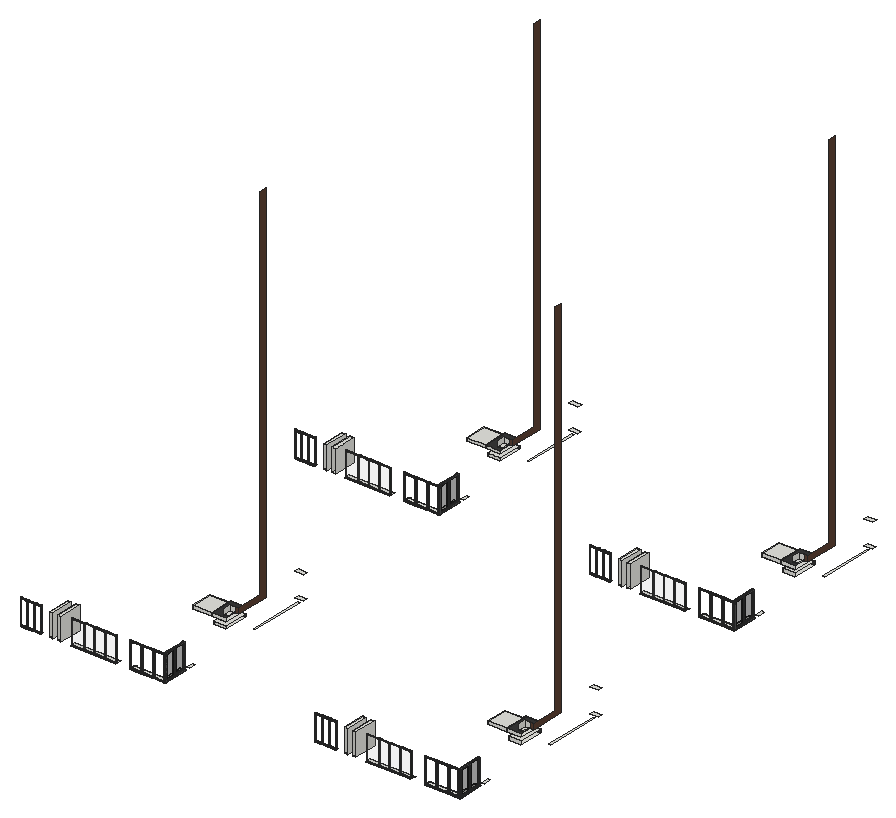
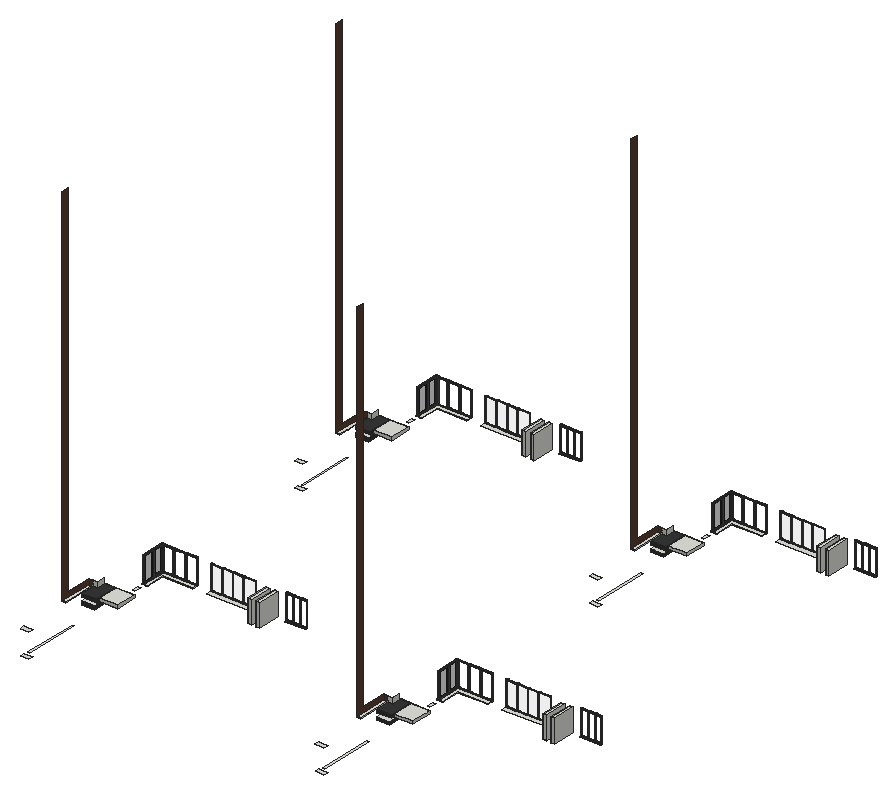
# SketchUp Ruby script. Lengths in inches.
U = 1.inch
M = Sketchup.active_model
def pt(a) = Geom::Point3d.new(a.map { |v| v * U })
def face(e, loops, mat)
  f = e.add_face(loops[0].map { |a| pt(a) })
  loops[1..].each { |l| e.add_face(l.map { |a| pt(a) }).erase! }
  f.material = f.back_material = mat if mat
  f
end
# faces: each face lists its corners as indices into pts; further lists are holes
def faces(e, pts, list, mat = nil) = list.each { |f| face(e, (f[0].is_a?(Array) ? f : [f]).map { |l| l.map { |i| pts[i] } }, mat) }
# xy, xz, yz: faces in a plane at the given z, y or x. An outline is a flat list of corners, or four numbers for a rectangle; further outlines are holes
def ring(l) = l.size == 4 ? [[l[0], l[1]], [l[2], l[1]], [l[2], l[3]], [l[0], l[3]]] : l.each_slice(2).to_a
def flat(e, list, mat, &to3) = list.each { |f| face(e, (f[0].is_a?(Array) ? f : [f]).map { |l| ring(l).map { |u, v| to3.(u, v) } }, mat) }
def xy(e, z, list, mat = nil) = flat(e, list, mat) { |x, y| [x, y, z] }
def xz(e, y, list, mat = nil) = flat(e, list, mat) { |x, z| [x, y, z] }
def yz(e, x, list, mat = nil) = flat(e, list, mat) { |y, z| [x, y, z] }
def lines(e, pts, list) = list.each { |a, b| e.add_line(pt(pts[a]), pt(pts[b])) }
# prism: a flat outline (further loops are holes) pulled along v
def prism(e, loops, v, mat = nil)
  f = face(e, loops, mat); d = Geom::Vector3d.new(v.map { |x| x * U })
  f.pushpull(f.normal.samedirection?(d) ? d.length : -d.length)
end
def box(e, o, s, mat = nil) = prism(e, [[o, [o[0] + s[0], o[1], o[2]], [o[0] + s[0], o[1] + s[1], o[2]], [o[0], o[1] + s[1], o[2]]]], [0, 0, s[2]], mat)
def at(x, y, z, deg = 0) = Geom::Transformation.translation(pt([x, y, z])) * Geom::Transformation.rotation(ORIGIN, Z_AXIS, deg.degrees)
def axes(o, x, y, z) = Geom::Transformation.new([*x, 0, *y, 0, *z, 0, *pt(o).to_a, 1])
def part(name) = M.definitions.add(name)
# library, detail: a bought-in or finely detailed component or shape, given as its bounding box
def library(name, o, s) = part(name).tap { |d| box(d.entities, o, s) }
def detail(e, o, s) = box(e.add_group.entities, o, s)
def put(e, d, t, mat = nil) = e.add_instance(d, t).tap { |i| i.material = mat if mat }
def group(e, t, mat = nil) = e.add_group.tap { |g| g.transformation = t; g.material = mat if mat }.entities
root = M.entities
M.materials.add("Glass_Tinted_Gray").color = [0, 0, 0]
M.materials["Glass_Tinted_Gray"].alpha = 0.125
M.materials.add("Glazing").color = [128, 128, 128]
M.materials["Glazing"].alpha = 0.05
M.materials.add("Powdercoating").color = [41, 44, 40]
M.materials.add("Wine2").color = [0, 0, 0]
M.materials["Wine2"].alpha = 0
M.materials.add("[0130_Gainsboro]").color = [39, 45, 50]
M.materials.add("[0135_DarkGray]").color = [81, 81, 81]
M.materials.add("[Granite Brown]1").color = [89, 63, 50]
M.materials.add("[Mirror 02]").color = [229, 229, 229]
M.materials.add("[Slate Light Tile]").color = [54, 54, 54]
M.materials.add("[Terrazzo Light Blue]").color = [196, 214, 227]
c1 = part("Framed glazing panel")
xy(c1.entities,0,[[0,-0.98,43.07,0],[0,0,43.07,1.4]],"[0130_Gainsboro]")
xy(c1.entities,0.3,[[0.3,-1.43,42.77,-0.98]],"[0130_Gainsboro]")
xy(c1.entities,2.95,[[2.95,-1.43,40.12,-0.63],[2.95,-0.63,40.12,0],[2.95,0,40.12,0.64],[2.95,0.64,40.12,1.4]],"[0130_Gainsboro]")
xy(c1.entities,3.54,[[3.54,-0.63,39.53,0],[3.54,0,39.53,0.64]],"[0130_Gainsboro]")
xy(c1.entities,111.8125,[[3.54,-0.63,39.53,0],[3.54,0,39.53,0.64]],"[0130_Gainsboro]")
xy(c1.entities,112.4,[[2.95,-1.43,40.12,-0.63],[2.95,-0.63,40.12,0],[2.95,0,40.12,0.64],[2.95,0.64,40.12,1.4]],"[0130_Gainsboro]")
xy(c1.entities,115.05,[[0.3,-1.43,42.77,-0.98]],"[0130_Gainsboro]")
xy(c1.entities,115.35,[[0,-0.98,43.07,0],[0,0,43.07,1.4]],"[0130_Gainsboro]")
xz(c1.entities,-1.43,[[[0.3,0.3,42.77,115.05],[2.95,2.95,40.12,112.4]]],"[0130_Gainsboro]")
xz(c1.entities,-0.98,[[[0,0,43.07,115.35],[0.3,0.3,42.77,115.05]]],"[0130_Gainsboro]")
xz(c1.entities,-0.63,[[[2.95,2.95,40.12,112.4],[3.54,3.54,39.53,111.8125]]],"[0130_Gainsboro]")
xz(c1.entities,0,[[3.54,3.54,39.53,111.8125]],"Wine2")
xz(c1.entities,0,[[[0,0,43.07,115.35],[2.95,2.95,40.12,112.4]],[[2.95,2.95,40.12,112.4],[3.54,3.54,39.53,111.8125]]],"[0130_Gainsboro]")
xz(c1.entities,0.64,[[[2.95,2.95,40.12,112.4],[3.54,3.54,39.53,111.8125]]],"[0130_Gainsboro]")
xz(c1.entities,1.4,[[[0,0,43.07,115.35],[2.95,2.95,40.12,112.4]]],"[0130_Gainsboro]")
yz(c1.entities,0,[[-0.98,0,0,115.35],[0,0,1.4,115.35]],"[0130_Gainsboro]")
yz(c1.entities,0.3,[[-1.43,0.3,-0.98,115.05]],"[0130_Gainsboro]")
yz(c1.entities,2.95,[[-1.43,2.95,-0.63,112.4],[-0.63,2.95,0,112.4],[0,2.95,0.64,112.4],[0.64,2.95,1.4,112.4]],"[0130_Gainsboro]")
yz(c1.entities,3.54,[[-0.63,3.54,0,111.8125],[0,3.54,0.64,111.8125]],"[0130_Gainsboro]")
yz(c1.entities,39.53,[[-0.63,3.54,0,111.8125],[0,3.54,0.64,111.8125]],"[0130_Gainsboro]")
yz(c1.entities,40.12,[[-1.43,2.95,-0.63,112.4],[-0.63,2.95,0,112.4],[0,2.95,0.64,112.4],[0.64,2.95,1.4,112.4]],"[0130_Gainsboro]")
yz(c1.entities,42.77,[[-1.43,0.3,-0.98,115.05]],"[0130_Gainsboro]")
yz(c1.entities,43.07,[[-0.98,0,0,115.35],[0,0,1.4,115.35]],"[0130_Gainsboro]")
c2 = part("Glazed panel assembly")
put(c2.entities,c1,axes([90.57,1.43,0],[1.05148,0,0],[0,1,0],[0,0,1]))
put(c2.entities,c1,axes([0,1.43,0],[1.05148,0,0],[0,1,0],[0,0,1]))
put(c2.entities,c1,axes([45.29,1.43,0],[1.05148,0,0],[0,1,0],[0,0,1]))
c3 = part("PENTEK_RP Fineline 50S_Sliding_DoorCase_E1")
box(c3.entities,[0,0,0],[1.51,3.66,99.27],"[0135_DarkGray]")
c4 = part("PENTEK_RP Fineline 50S_SlidingDooe_Case_E2")
box(c4.entities,[0,0,0],[96.25,3.66,1.51],"[0135_DarkGray]")
c5 = part("pentek_RP Fineline 50S_SlidingDoor_Case")
put(c5.entities,c3,at(97.76,0,0))
put(c5.entities,c4,at(1.51,0,0))
put(c5.entities,c3,at(0,0,0))
put(c5.entities,c4,at(1.51,0,97.76))
c6 = part("PENTEK_RP Fineline 50S_SlidingDoor_GlazingBead_2")
box(c6.entities,[0,0,0],[0.56,0.59,94.39],"[0135_DarkGray]")
c7 = part("PENTEK_RP Fineline 50S_SlidingDoor_Glass")
box(c7.entities,[0,0,0],[46.58,0.16,94.39],"Glass_Tinted_Gray")
c8 = part("PENTEK_RP Fineline 50S_SlidingDoor_GlazingBead")
box(c8.entities,[0,0,0],[45.47,0.59,0.56],"[0135_DarkGray]")
c9 = part("PENTEK_RP Fineline 50S_SlidingDoor_Leaf_E1")
xy(c9.entities,0,[[0,0,0.93,1.97],[0.93,1.57,1.49,1.97]],"[0135_DarkGray]")
xy(c9.entities,96.25,[[0,0,0.93,0,0.93,1.57,1.49,1.57,1.49,1.97,0,1.97]],"[0135_DarkGray]")
xz(c9.entities,0,[[0,0,0.93,96.25]],"[0135_DarkGray]")
xz(c9.entities,1.57,[[0.93,0,1.49,95.32],[0.93,95.32,1.49,96.25]],"[0135_DarkGray]")
xz(c9.entities,1.97,[[0,0,1.49,96.25]],"[0135_DarkGray]")
yz(c9.entities,0,[[0,0,1.97,96.25]],"[0135_DarkGray]")
yz(c9.entities,0.93,[[0,0,1.57,0.93],[0,0.93,1.57,95.32],[0,95.32,1.57,96.25]],"[0135_DarkGray]")
yz(c9.entities,1.49,[[1.57,0,1.97,95.32],[1.57,95.32,1.97,96.25]],"[0135_DarkGray]")
c10 = part("PENTEK_RP Fineline 50S_SlidingDoor_Leaf_E2")
xy(c10.entities,0,[[0,0,0,1.57,0.56,1.57,0.56,1.97,46.02,1.97,46.02,1.57,46.58,1.57,46.58,0]],"[0135_DarkGray]")
xy(c10.entities,0.93,[[0,0,46.58,1.57]],"[0135_DarkGray]")
xy(c10.entities,1.49,[[0.56,1.57,46.02,1.97]],"[0135_DarkGray]")
xz(c10.entities,0,[[0,0,46.58,0.93]],"[0135_DarkGray]")
xz(c10.entities,1.57,[[0,0,0.56,0.93],[46.02,0,46.58,0.93],[0.56,0.93,46.02,1.49]],"[0135_DarkGray]")
xz(c10.entities,1.97,[[0.56,0,46.02,1.49]],"[0135_DarkGray]")
yz(c10.entities,0,[[0,0,1.57,0.93]],"[0135_DarkGray]")
yz(c10.entities,0.56,[[1.57,0,1.97,0.93],[1.57,0.93,1.97,1.49]],"[0135_DarkGray]")
yz(c10.entities,46.02,[[1.57,0,1.97,0.93],[1.57,0.93,1.97,1.49]],"[0135_DarkGray]")
yz(c10.entities,46.58,[[0,0,1.57,0.93]],"[0135_DarkGray]")
c11 = part("PENTEK_RP Fineline S_SlidingDoor_Leaf1")
put(c11.entities,c6,at(0.93,0,0.93))
put(c11.entities,c6,at(46.96,0,0.93))
put(c11.entities,c7,at(1.49,1.42,0.93))
put(c11.entities,c8,at(1.49,0,0.93))
put(c11.entities,c7,at(1.49,0.59,0.93),"[Terrazzo Light Blue]")
put(c11.entities,c9,at(0,0,0))
put(c11.entities,c9,axes([48.44,0,0],[-1,0,0],[0,1,0],[0,0,1]))
put(c11.entities,c10,axes([0.93,0,96.25],[1,0,0],[0,1,0],[0,0,-1]))
put(c11.entities,c10,at(0.93,0,0))
put(c11.entities,c8,at(1.49,0,94.77))
c12 = part("PENTEK_RP Fineline 50S_SlidingDoor_Leaf2")
put(c12.entities,c7,at(1.49,1.42,0.93))
put(c12.entities,c8,at(1.49,0,94.77))
put(c12.entities,c6,at(46.96,0,0.93))
put(c12.entities,c7,at(1.49,0.59,0.93),"[Mirror 02]")
put(c12.entities,c6,at(0.93,0,0.93))
put(c12.entities,c9,at(0,0,0))
put(c12.entities,c9,axes([48.44,0,0],[-1,0,0],[0,1,0],[0,0,1]))
put(c12.entities,c8,at(1.49,0,0.93))
put(c12.entities,c10,axes([0.93,0,96.25],[1,0,0],[0,1,0],[0,0,-1]))
put(c12.entities,c10,at(0.93,0,0))
c13 = part("PENTEK - Slimmest Steel Sliding Door / Window\#1")
put(c13.entities,c5,at(0,-1.88,-0.09))
put(c13.entities,c11,at(1.51,-2.27,1.42))
put(c13.entities,c12,at(49.32,-0.3,1.42))
c14 = part("Group\#15")
xy(c14.entities,0,[[0,-55.94,0.71,45.94]])
xy(c14.entities,0.2,[[0,-55.94,0.47,45.94],[0.47,45.94,0.71,46.42]])
xy(c14.entities,2.36,[[0.47,-55.94,0.71,46.42]])
xz(c14.entities,-55.94,[[0,0,0.71,0,0.71,2.36,0.47,2.36,0.47,0.2,0,0.2]])
xz(c14.entities,45.94,[[0,0,0.71,0.2]])
xz(c14.entities,46.42,[[0.47,0.2,0.71,2.36]])
yz(c14.entities,0,[[-55.94,0,45.94,0.2]])
yz(c14.entities,0.47,[[-55.94,0.2,46.42,2.36]])
yz(c14.entities,0.71,[[-55.94,0,45.94,0,45.94,0.2,46.42,0.2,46.42,2.36,-55.94,2.36]])
c15 = part("Group\#7")
xy(c15.entities,0,[[0,-59.09,0.71,45.94]])
xy(c15.entities,0.2,[[0,-59.09,0.47,45.94],[0.47,45.94,0.71,46.42]])
xy(c15.entities,2.36,[[0.47,-59.09,0.71,46.42]])
xz(c15.entities,-59.09,[[0,0,0.71,0,0.71,2.36,0.47,2.36,0.47,0.2,0,0.2]])
xz(c15.entities,45.94,[[0,0,0.71,0.2]])
xz(c15.entities,46.42,[[0.47,0.2,0.71,2.36]])
yz(c15.entities,0,[[-59.09,0,45.94,0.2]])
yz(c15.entities,0.47,[[-59.09,0.2,46.42,2.36]])
yz(c15.entities,0.71,[[-59.09,0,45.94,0,45.94,0.2,46.42,0.2,46.42,2.36,-59.09,2.36]])
c16 = part("Group\#16")
prism(c16.entities,[[[0.47,-56.18,0.2],[0,-56.18,0.2],[0,-56.18,0],[0.71,-56.18,0],[0.71,-56.18,2.36],[0.47,-56.18,2.36]]],[0,28.68,0])
c17 = part("Group\#10")
box(c17.entities,[-0.73,0,0],[27.99,0.55,102.05])
c18 = part("Group\#18")
xy(c18.entities,0,[[0.47,-56.18,0.47,-55.47,0,-55.47,0,-28.21,1.18,-28.21,1.18,-56.18]])
xy(c18.entities,0.2,[[0.71,-56.18,1.18,-28.21],[0,-55.47,0.47,-28.21],[0.47,-28.21,0.71,-27.74]])
xy(c18.entities,2.36,[[0.47,-56.18,0.71,-27.74]])
xz(c18.entities,-56.18,[[0.47,0,1.18,0,1.18,0.2,0.71,0.2,0.71,2.36,0.47,2.36]])
xz(c18.entities,-55.47,[[0,0,0.47,0.2]])
xz(c18.entities,-28.21,[[0,0,1.18,0.2]])
xz(c18.entities,-27.74,[[0.47,0.2,0.71,2.36]])
yz(c18.entities,0,[[-55.47,0,-28.21,0.2]])
yz(c18.entities,0.47,[[-56.18,0,-55.47,0.2],[-56.18,0.2,-27.74,2.36]])
yz(c18.entities,0.71,[[-56.18,0.2,-27.74,2.36]])
yz(c18.entities,1.18,[[-56.18,0,-28.21,0.2]])
c19 = part("Group\#34")
xy(c19.entities,0,[[-20.45,0,7.76,1.22]])
xy(c19.entities,0.06,[[-20.39,0.06,7.7,1.22]])
xy(c19.entities,0.47,[[-19.98,0,7.28,0.06]])
xy(c19.entities,101.89,[[-19.98,0,7.28,0.06]])
xy(c19.entities,102.3,[[-20.39,0.06,7.7,1.22]])
xy(c19.entities,102.36,[[-20.45,0,7.76,1.22]])
xz(c19.entities,0,[[[-20.45,0,7.76,102.36],[-19.98,0.47,7.28,101.89]]])
xz(c19.entities,0.06,[[[-20.39,0.06,7.7,102.3],[-19.98,0.47,7.28,101.89]]])
xz(c19.entities,1.22,[[[-20.45,0,7.76,102.36],[-20.39,0.06,7.7,102.3]]])
yz(c19.entities,-20.45,[[0,0,1.22,102.36]])
yz(c19.entities,-20.39,[[0.06,0.06,1.22,102.3]])
yz(c19.entities,-19.98,[[0,0.47,0.06,101.89]])
yz(c19.entities,7.28,[[0,0.47,0.06,101.89]])
yz(c19.entities,7.7,[[0.06,0.06,1.22,102.3]])
yz(c19.entities,7.76,[[0,0,1.22,102.36]])
c20 = part("Group\#6")
put(c20.entities,c14,axes([27.97,0,7.875],[1,0,0],[0,0,-1],[0,1,0]),"Powdercoating")
put(c20.entities,c15,axes([0.71,0,6.8],[-1,0,0],[0,0,-0.97687],[0,1,0]),"Powdercoating")
put(c20.entities,c16,axes([-27.5,0,-38.07],[0,0,-1],[-1,0,0],[0,1,0]),"Powdercoating")
put(c20.entities,c17,at(1.12,0.35,-38.39),"Glazing")
put(c20.entities,c18,axes([-27.5,0,63.35],[0,0,1],[-1,0,0],[0,1,0]),"Powdercoating")
put(c20.entities,c19,at(20.6875,1.0625,-38.54),"Powdercoating")
c21 = part("Sliding door assembly")
put(c21.entities,c20,at(-1.18,4.5,38.86))
g1 = group(c21.entities,at(84.74,4.5,38.86))
put(g1,c14,axes([-27.97,0,7.875],[-1,0,0],[0,0,-1],[0,1,0]),"Powdercoating")
put(g1,c15,axes([-0.71,0,6.8],[1,0,0],[0,0,-0.97687],[0,1,0]),"Powdercoating")
put(g1,c16,axes([27.5,0,-38.07],[0,0,-1],[1,0,0],[0,1,0]),"Powdercoating")
put(g1,c17,axes([-1.12,0.35,-38.39],[-1,0,0],[0,1,0],[0,0,1]),"Glazing")
put(g1,c18,axes([27.5,0,63.35],[0,0,1],[1,0,0],[0,1,0]),"Powdercoating")
put(g1,c19,axes([-20.6875,1.0625,-38.54],[-1,0,0],[0,1,0],[0,0,1]),"Powdercoating")
g2 = group(c21.entities,at(56.0625,4.5,38.86))
put(g2,c14,axes([-27.97,0,7.875],[-1,0,0],[0,0,-1],[0,1,0]),"Powdercoating")
put(g2,c16,axes([27.5,0,-38.07],[0,0,-1],[1,0,0],[0,1,0]),"Powdercoating")
put(g2,c17,axes([-1.12,0.35,-38.39],[-1,0,0],[0,1,0],[0,0,1]),"Glazing")
put(g2,c18,axes([27.5,0,63.35],[0,0,1],[1,0,0],[0,1,0]),"Powdercoating")
put(g2,c19,axes([-20.6875,1.0625,-38.54],[-1,0,0],[0,1,0],[0,0,1]),"Powdercoating")
g3 = group(g2,at(-0.71,0,6.8),"Powdercoating")
xy(g3,-45.34,[[0.47,0.2,0.71,2.36]])
xy(g3,-44.88,[[0,0,0.71,0.2]])
xy(g3,57.73,[[0,0,0.71,0,0.71,2.36,0.47,2.36,0.47,0.2,0,0.2]])
xz(g3,0,[[0,-44.88,0.71,57.73]])
xz(g3,0.2,[[0.47,-45.34,0.71,-44.88],[0,-44.88,0.47,57.73]])
xz(g3,2.36,[[0.47,-45.34,0.71,57.73]])
yz(g3,0,[[0,-44.88,0.2,57.73]])
yz(g3,0.47,[[0.2,-45.34,2.36,57.73]])
yz(g3,0.71,[[0.2,-45.34,2.36,-45.34,2.36,57.73,0,57.73,0,-44.88,0.2,-44.88]])
put(c21.entities,c20,axes([-33.94,4.5,38.86],[1.14218,0,0],[0,1,0],[0,0,1]))
c22 = part("sliding door")
put(c22.entities,c21,at(0,-4.5,-0.08))
prism(root,[[[2132.0625,1799.9375,145.375],[1985.38,1799.9375,145.375],[1985.38,1822.9375,145.375],[2109.0625,1822.9375,145.375],[2109.0625,1902.66,145.375],[2132.0625,1902.66,145.375]]],[0,0,1.75])
prism(root,[[[913.875,1799.9375,145.375],[767.19,1799.9375,145.375],[767.19,1822.9375,145.375],[890.875,1822.9375,145.375],[890.875,1902.66,145.375],[913.875,1902.66,145.375]]],[0,0,1.75])
prism(root,[[[2132.0625,3214.625,145.375],[1985.38,3214.625,145.375],[1985.38,3237.625,145.375],[2109.0625,3237.625,145.375],[2109.0625,3317.34,145.375],[2132.0625,3317.34,145.375]]],[0,0,1.75])
prism(root,[[[913.875,3214.625,145.375],[767.19,3214.625,145.375],[767.19,3237.625,145.375],[890.875,3237.625,145.375],[890.875,3317.34,145.375],[913.875,3317.34,145.375]]],[0,0,1.75])
xy(root,145.375,[[319.53,1799.9375,399.88,1807.625],[523.04,1799.9375,709.87,1822.9375],[1537.72,1799.9375,1618.07,1807.625],[1741.23,1799.9375,1928.05,1822.9375],[902.375,1926.07,913.875,1953.7],
  [2120.5625,1926.07,2132.0625,1953.7],[913.875,2258.18,921.125,2483.21],[2132.0625,2258.18,2139.3125,2483.21],[890.875,2497.47,927.0625,2514.84],[2109.0625,2497.47,2145.25,2514.84],
  [319.53,3214.625,399.88,3222.3125],[523.04,3214.625,709.87,3237.625],[1537.72,3214.625,1618.07,3222.3125],[1741.23,3214.625,1928.05,3237.625],[902.375,3340.76,913.875,3368.39],
  [2120.5625,3340.76,2132.0625,3368.39],[913.875,3672.87,921.125,3897.9],[2132.0625,3672.87,2139.3125,3897.9],[890.875,3912.16,927.0625,3929.52],[2109.0625,3912.16,2145.25,3929.52]])
xy(root,145.8125,[[434.43,1799.9375,450.49,1893.25],[1652.62,1799.9375,1668.68,1893.25],[434.43,3214.625,450.49,3307.9375],[1652.62,3214.625,1668.68,3307.9375]])
xy(root,147.29,[[467.98,1799.9375,483.79,1893.25],[1686.17,1799.9375,1701.98,1893.25],[467.98,3214.625,483.79,3307.9375],[1686.17,3214.625,1701.98,3307.9375]])
xy(root,206.6875,[[861.3125,2113.57,913.875,2213.62],[2079.5,2113.57,2132.0625,2213.62],[861.3125,3528.25,913.875,3628.31],[2079.5,3528.25,2132.0625,3628.31]])
xy(root,220.18,[[861.3125,2113.57,913.875,2213.62],[2079.5,2113.57,2132.0625,2213.62],[861.3125,3528.25,913.875,3628.31],[2079.5,3528.25,2132.0625,3628.31]])
xy(root,234.11,[[776.875,2113.57,853.875,2200.82],[853.875,2113.57,913.875,2213.62],[1995.0625,2113.57,2072.0625,2200.82],[2072.0625,2113.57,2132.0625,2213.62],[776.875,3528.25,853.875,3615.5],
  [853.875,3528.25,913.875,3628.31],[1995.0625,3528.25,2072.0625,3615.5],[2072.0625,3528.25,2132.0625,3628.31]])
xy(root,240.11,[[467.98,1799.9375,483.79,1893.25],[1686.17,1799.9375,1701.98,1893.25],[467.98,3214.625,483.79,3307.9375],[1686.17,3214.625,1701.98,3307.9375]])
xy(root,240.875,[[434.43,1799.9375,450.49,1893.25],[1652.62,1799.9375,1668.68,1893.25],[434.43,3214.625,450.49,3307.9375],[1652.62,3214.625,1668.68,3307.9375]])
xy(root,245.15,[[890.875,2497.47,927.75,2514.84],[2109.0625,2497.47,2145.9375,2514.84],[890.875,3912.16,927.75,3929.52],[2109.0625,3912.16,2145.9375,3929.52]])
xy(root,246.61,[[776.875,2113.57,853.875,2200.82],[1995.0625,2113.57,2072.0625,2200.82],[776.875,3528.25,853.875,3615.5],[1995.0625,3528.25,2072.0625,3615.5]])
xy(root,246.61,[[853.875,2113.57,913.875,2213.62],[2072.0625,2113.57,2132.0625,2213.62],[853.875,3528.25,913.875,3628.31],[2072.0625,3528.25,2132.0625,3628.31]],"[Slate Light Tile]")
xy(root,248.9375,[[894.3125,2124.51,913.875,2156.01],[2112.5,2124.51,2132.0625,2156.01],[913.875,2156.01,930.75,2295.875],[2132.0625,2156.01,2148.9375,2295.875],[894.3125,3539.2,913.875,3570.7],
  [2112.5,3539.2,2132.0625,3570.7],[913.875,3570.7,930.75,3710.5625],[2132.0625,3570.7,2148.9375,3710.5625]])
xz(root,1893.25,[[434.43,145.8125,450.49,240.875],[1652.62,145.8125,1668.68,240.875],[467.98,147.29,483.79,240.11],[1686.17,147.29,1701.98,240.11]])
xz(root,2113.57,[[861.3125,206.6875,913.875,220.18],[2079.5,206.6875,2132.0625,220.18],[776.875,234.11,853.875,246.61],[853.875,234.11,913.875,246.61],[1995.0625,234.11,2072.0625,246.61],
  [2072.0625,234.11,2132.0625,246.61]])
xz(root,2124.51,[[894.3125,248.9375,913.875,252],[2112.5,248.9375,2132.0625,252]])
xz(root,2156.01,[[894.3125,248.9375,913.875,271.5],[2112.5,248.9375,2132.0625,271.5]])
xz(root,2156.01,[[913.875,248.9375,930.75,271.5],[2132.0625,248.9375,2148.9375,271.5]],"[Granite Brown]1")
xz(root,2200.82,[[776.875,234.11,853.875,246.61],[1995.0625,234.11,2072.0625,246.61]])
xz(root,2213.62,[[861.3125,206.6875,913.875,220.18],[2079.5,206.6875,2132.0625,220.18],[853.875,234.11,913.875,246.61],[2072.0625,234.11,2132.0625,246.61]],"[Slate Light Tile]")
xz(root,2295.875,[[913.875,248.9375,930.75,252],[2132.0625,248.9375,2148.9375,252]])
xz(root,3307.9375,[[434.43,145.8125,450.49,240.875],[1652.62,145.8125,1668.68,240.875],[467.98,147.29,483.79,240.11],[1686.17,147.29,1701.98,240.11]])
xz(root,3528.25,[[861.3125,206.6875,913.875,220.18],[2079.5,206.6875,2132.0625,220.18],[776.875,234.11,853.875,246.61],[853.875,234.11,913.875,246.61],[1995.0625,234.11,2072.0625,246.61],
  [2072.0625,234.11,2132.0625,246.61]])
xz(root,3539.2,[[894.3125,248.9375,913.875,252],[2112.5,248.9375,2132.0625,252]])
xz(root,3570.7,[[894.3125,248.9375,913.875,271.5],[2112.5,248.9375,2132.0625,271.5]])
xz(root,3570.7,[[913.875,248.9375,930.75,271.5],[2132.0625,248.9375,2148.9375,271.5]],"[Granite Brown]1")
xz(root,3615.5,[[776.875,234.11,853.875,246.61],[1995.0625,234.11,2072.0625,246.61]])
xz(root,3628.31,[[861.3125,206.6875,913.875,220.18],[2079.5,206.6875,2132.0625,220.18],[853.875,234.11,913.875,246.61],[2072.0625,234.11,2132.0625,246.61]],"[Slate Light Tile]")
xz(root,3710.5625,[[913.875,248.9375,930.75,252],[2132.0625,248.9375,2148.9375,252]])
yz(root,434.43,[[1799.9375,145.8125,1893.25,240.875],[3214.625,145.8125,3307.9375,240.875]])
yz(root,450.49,[[1799.9375,145.8125,1893.25,240.875],[3214.625,145.8125,3307.9375,240.875]])
yz(root,467.98,[[1799.9375,147.29,1893.25,240.11],[3214.625,147.29,3307.9375,240.11]])
yz(root,483.79,[[1799.9375,147.29,1893.25,240.11],[3214.625,147.29,3307.9375,240.11]])
yz(root,776.875,[[2113.57,234.11,2200.82,246.61],[3528.25,234.11,3615.5,246.61]])
yz(root,853.875,[[2113.57,234.11,2200.82,246.61],[2200.82,234.11,2213.62,246.61],[3528.25,234.11,3615.5,246.61],[3615.5,234.11,3628.31,246.61]],"[Slate Light Tile]")
yz(root,861.3125,[[2113.57,206.6875,2213.62,220.18],[3528.25,206.6875,3628.31,220.18]],"[Slate Light Tile]")
yz(root,894.3125,[[2124.51,248.9375,2156.01,271.5],[3539.2,248.9375,3570.7,271.5]])
yz(root,913.875,[[2124.51,248.9375,2156.01,252],[2156.01,248.9375,2258.18,252],[2258.18,248.9375,2295.875,252],[3539.2,248.9375,3570.7,252],[3570.7,248.9375,3672.87,252],
  [3672.87,248.9375,3710.5625,252]])
yz(root,930.75,[[2156.01,248.9375,2295.875,248.9375,2295.875,1764,2266.33,1764,2266.33,271.5,2156.01,271.5],[3570.7,248.9375,3710.5625,248.9375,3710.5625,1764,3681.01,1764,3681.01,271.5,3570.7,271.5]],"[Granite Brown]1")
yz(root,1652.62,[[1799.9375,145.8125,1893.25,240.875],[3214.625,145.8125,3307.9375,240.875]])
yz(root,1668.68,[[1799.9375,145.8125,1893.25,240.875],[3214.625,145.8125,3307.9375,240.875]])
yz(root,1686.17,[[1799.9375,147.29,1893.25,240.11],[3214.625,147.29,3307.9375,240.11]])
yz(root,1701.98,[[1799.9375,147.29,1893.25,240.11],[3214.625,147.29,3307.9375,240.11]])
yz(root,1995.0625,[[2113.57,234.11,2200.82,246.61],[3528.25,234.11,3615.5,246.61]])
yz(root,2072.0625,[[2113.57,234.11,2200.82,246.61],[2200.82,234.11,2213.62,246.61],[3528.25,234.11,3615.5,246.61],[3615.5,234.11,3628.31,246.61]],"[Slate Light Tile]")
yz(root,2079.5,[[2113.57,206.6875,2213.62,220.18],[3528.25,206.6875,3628.31,220.18]],"[Slate Light Tile]")
yz(root,2112.5,[[2124.51,248.9375,2156.01,271.5],[3539.2,248.9375,3570.7,271.5]])
yz(root,2132.0625,[[2124.51,248.9375,2156.01,252],[2156.01,248.9375,2258.18,252],[2258.18,248.9375,2295.875,252],[3539.2,248.9375,3570.7,252],[3570.7,248.9375,3672.87,252],
  [3672.87,248.9375,3710.5625,252]])
yz(root,2148.9375,[[2156.01,248.9375,2295.875,248.9375,2295.875,1764,2266.33,1764,2266.33,271.5,2156.01,271.5],[3570.7,248.9375,3710.5625,248.9375,3710.5625,1764,3681.01,1764,3681.01,271.5,3570.7,271.5]],"[Granite Brown]1")
put(root,c2,axes([1532.51,1799.9375,145.375],[0.62975,0,0],[0,1,0],[0,0,0.91782]))
put(root,c2,axes([314.33,1799.9375,145.375],[0.62975,0,0],[0,1,0],[0,0,0.91782]))
put(root,c2,axes([1532.51,3214.625,145.375],[0.62975,0,0],[0,1,0],[0,0,0.91782]))
put(root,c2,axes([314.33,3214.625,145.375],[0.62975,0,0],[0,1,0],[0,0,0.91782]))
put(root,c2,axes([1984.39,1799.9375,145.375],[1.09,0,0],[0,1,0],[0,0,0.91782]))
put(root,c2,axes([766.2,1799.9375,145.375],[1.09,0,0],[0,1,0],[0,0,0.91782]))
put(root,c2,axes([1984.39,3214.625,145.375],[1.09,0,0],[0,1,0],[0,0,0.91782]))
put(root,c2,axes([766.2,3214.625,145.375],[1.09,0,0],[0,1,0],[0,0,0.91782]))
put(root,c13,axes([2127.76,1799.9375,147.14],[0,1.02084,0],[-2.51374,0,0],[0,0,1.05725]))
put(root,c13,axes([909.57,1799.9375,147.14],[0,1.02084,0],[-2.51374,0,0],[0,0,1.05725]))
put(root,c13,axes([2127.76,3214.625,147.14],[0,1.02084,0],[-2.51374,0,0],[0,0,1.05725]))
put(root,c13,axes([909.57,3214.625,147.14],[0,1.02084,0],[-2.51374,0,0],[0,0,1.05725]))
put(root,c22,axes([1796.74,1799.9375,147.44],[1.54959,0,0],[0,1,0],[0,0,0.98]))
put(root,c22,axes([578.55,1799.9375,147.44],[1.54959,0,0],[0,1,0],[0,0,0.98]))
put(root,c22,axes([1796.74,3214.625,147.44],[1.54959,0,0],[0,1,0],[0,0,0.98]))
put(root,c22,axes([578.55,3214.625,147.44],[1.54959,0,0],[0,1,0],[0,0,0.98]))
